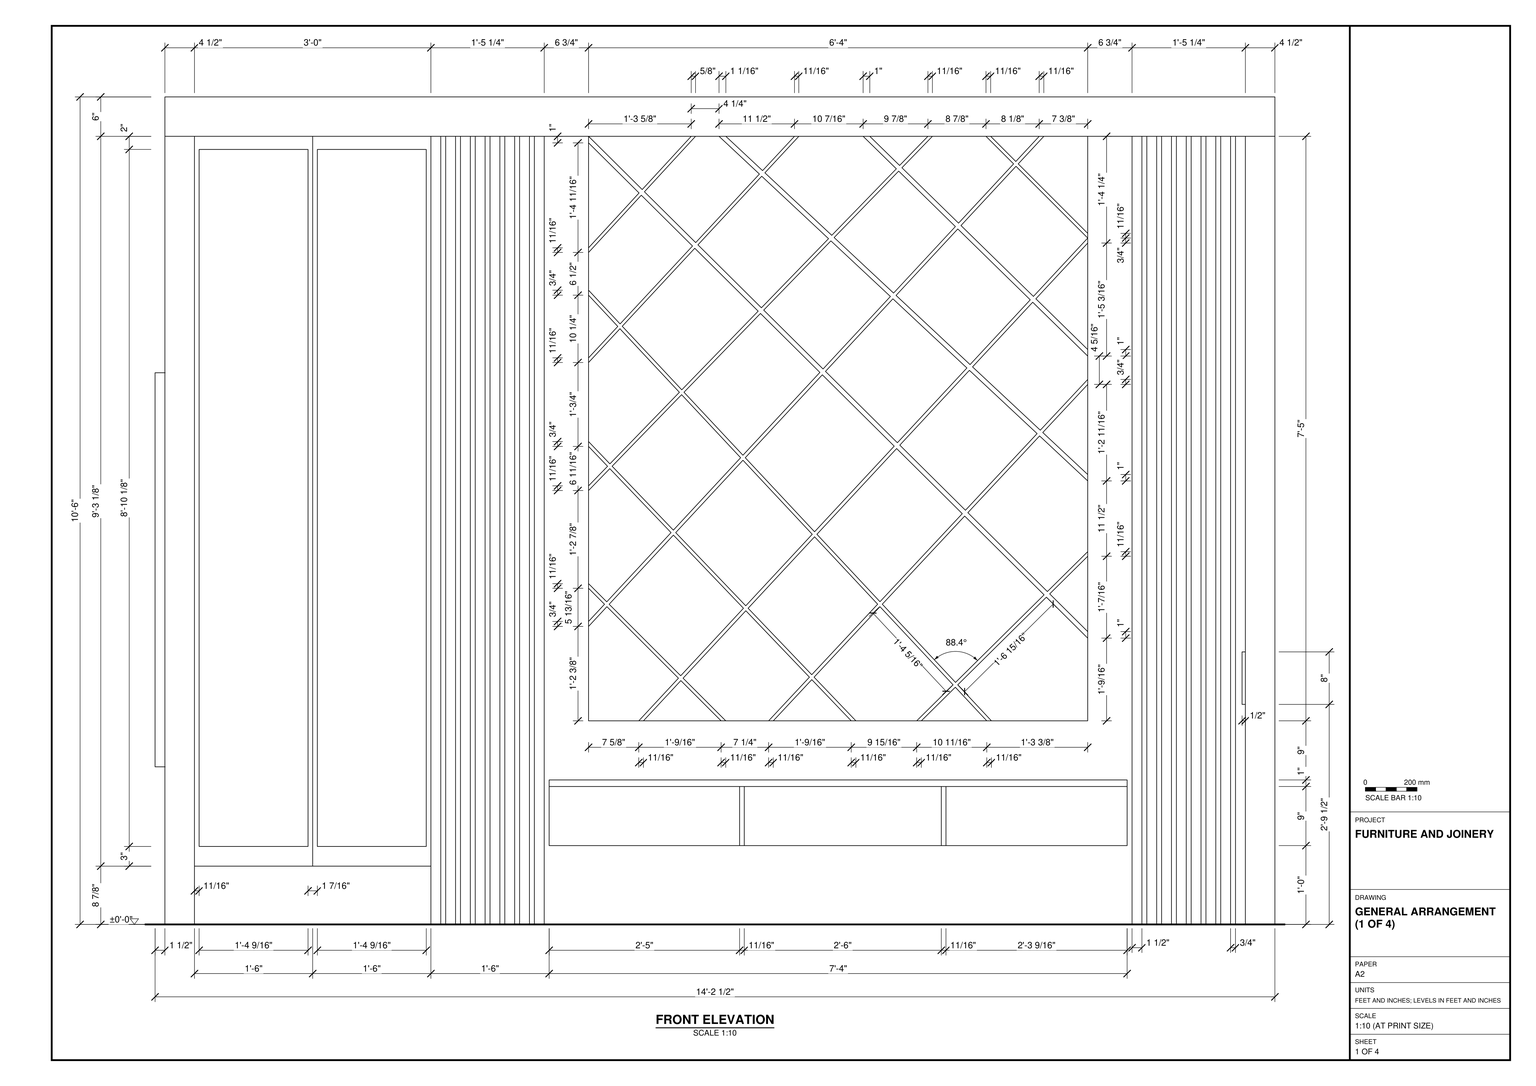
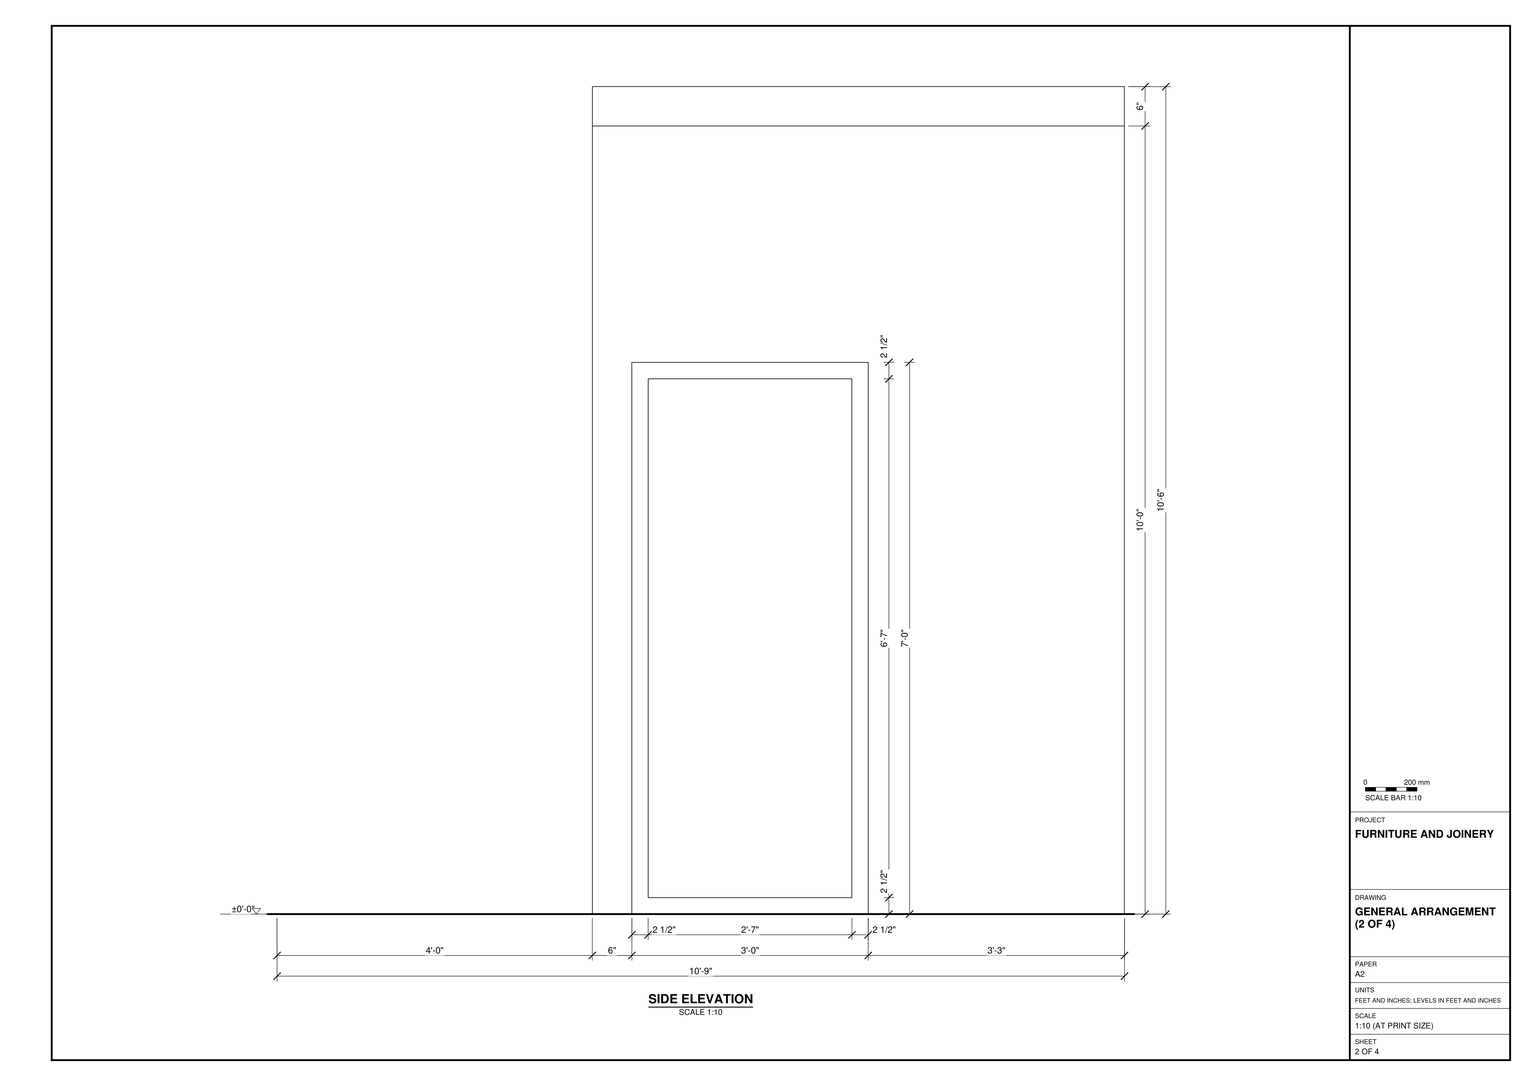
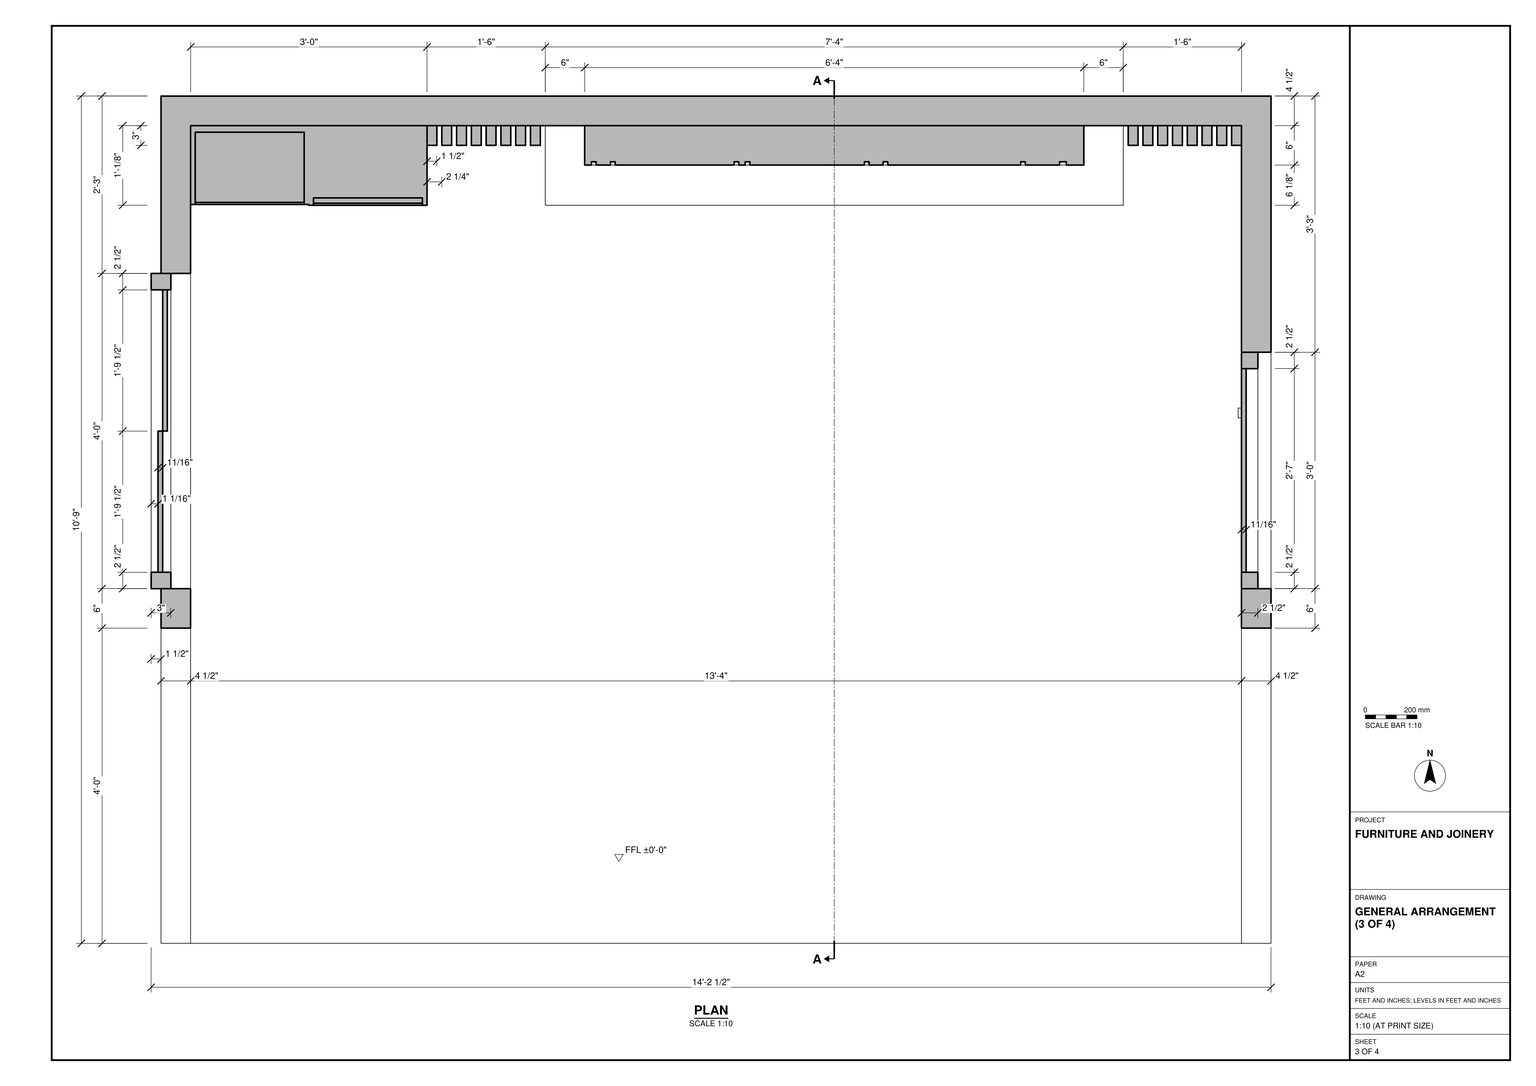
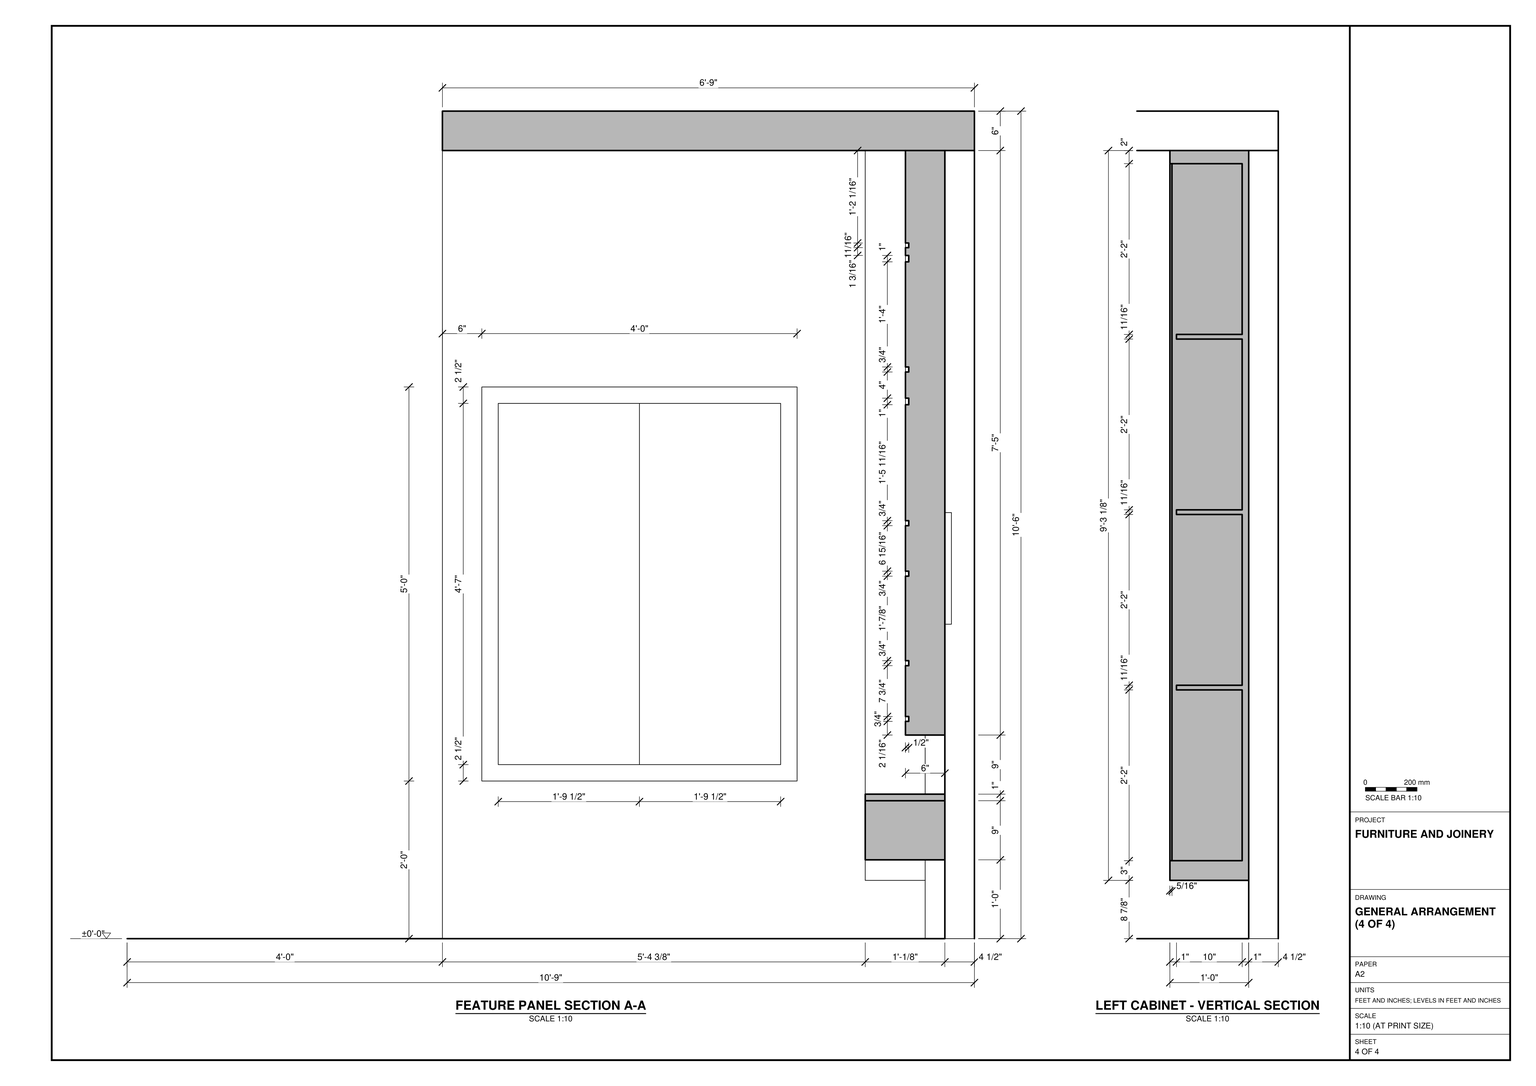
Build the feature-wall joinery and its surrounding room shell in SketchUp from task_files/diagram_01.pdf. Work in feet and inches. Set the finished floor at ±0'-0" and make the overall model 14'-2 1/2" wide, 10'-9" deep and 10'-6" high.

Use the plan to lay out the back wall and the two 4 1/2" thick side returns. Leave the front open, with the floor extending 4'-0" beyond the ends of the returns. Include the upper slab, the framed window in the left return and the framed door in the right return.

Facing the back wall, place the tall storage unit with paired inset fronts at the far left. Set out the central panel between the two bands of vertical slats. Follow the front elevation for the crossing diagonal lines, including where the diamonds are cut off at the panel edges. Below the panel, model the floating console with its thin top and three front sections. Use the plan to distinguish the projections of the panel, slats and storage units from the wall face.

Keep each shell element and each joinery piece in a separate group or component, and use components for repeated parts. Any decor or loose items shown may use suitable library components. Save one SketchUp model as output_files/feature_wall_with_built_in_storage_and_floating_console.skp.

# SketchUp Ruby script. Lengths in inches.
U = 1.inch
M = Sketchup.active_model
def pt(a) = Geom::Point3d.new(a.map { |v| v * U })
def face(e, loops, mat)
  f = e.add_face(loops[0].map { |a| pt(a) })
  loops[1..].each { |l| e.add_face(l.map { |a| pt(a) }).erase! }
  f.material = f.back_material = mat if mat
  f
end
# faces: each face lists its corners as indices into pts; further lists are holes
def faces(e, pts, list, mat = nil) = list.each { |f| face(e, (f[0].is_a?(Array) ? f : [f]).map { |l| l.map { |i| pts[i] } }, mat) }
# xy, xz, yz: faces in a plane at the given z, y or x. An outline is a flat list of corners, or four numbers for a rectangle; further outlines are holes
def ring(l) = l.size == 4 ? [[l[0], l[1]], [l[2], l[1]], [l[2], l[3]], [l[0], l[3]]] : l.each_slice(2).to_a
def flat(e, list, mat, &to3) = list.each { |f| face(e, (f[0].is_a?(Array) ? f : [f]).map { |l| ring(l).map { |u, v| to3.(u, v) } }, mat) }
def xy(e, z, list, mat = nil) = flat(e, list, mat) { |x, y| [x, y, z] }
def xz(e, y, list, mat = nil) = flat(e, list, mat) { |x, z| [x, y, z] }
def yz(e, x, list, mat = nil) = flat(e, list, mat) { |y, z| [x, y, z] }
def lines(e, pts, list) = list.each { |a, b| e.add_line(pt(pts[a]), pt(pts[b])) }
# prism: a flat outline (further loops are holes) pulled along v
def prism(e, loops, v, mat = nil)
  f = face(e, loops, mat); d = Geom::Vector3d.new(v.map { |x| x * U })
  f.pushpull(f.normal.samedirection?(d) ? d.length : -d.length)
end
def box(e, o, s, mat = nil) = prism(e, [[o, [o[0] + s[0], o[1], o[2]], [o[0] + s[0], o[1] + s[1], o[2]], [o[0], o[1] + s[1], o[2]]]], [0, 0, s[2]], mat)
def at(x, y, z, deg = 0) = Geom::Transformation.translation(pt([x, y, z])) * Geom::Transformation.rotation(ORIGIN, Z_AXIS, deg.degrees)
def axes(o, x, y, z) = Geom::Transformation.new([*x, 0, *y, 0, *z, 0, *pt(o).to_a, 1])
def part(name) = M.definitions.add(name)
# library, detail: a bought-in or finely detailed component or shape, given as its bounding box
def library(name, o, s) = part(name).tap { |d| box(d.entities, o, s) }
def detail(e, o, s) = box(e.add_group.entities, o, s)
def put(e, d, t, mat = nil) = e.add_instance(d, t).tap { |i| i.material = mat if mat }
def group(e, t, mat = nil) = e.add_group.tap { |g| g.transformation = t; g.material = mat if mat }.entities
root = M.entities
M.materials.add("Flooring Parquet Parallel E01 120cm").color = [119, 88, 63]
M.materials.add("Glass Yellow 001").color = [0, 0, 0]
M.materials["Glass Yellow 001"].alpha = 0.1
M.materials.add("Marble Beige 23-58 150cm").color = [206, 178, 147]
M.materials.add("Marble Black 01 150cm").color = [31, 31, 31]
M.materials.add("Metal Sandblasted Black 200cm").color = [86, 90, 95]
M.materials.add("Porcelain Poised Taupe Matte 001").color = [140, 135, 132]
M.materials.add("Wall Paint Fine Grain 01 Yellow 100cm").color = [207, 190, 139]
M.materials.add("Wood Tiles Dark Shiny 02 100cm").color = [42, 30, 20]
c1 = library("Group\#3",[0,-6,0],[76,6,89])
g1 = group(root,at(6,4.5,0))
xy(g1,0,[[0,-4.5,160,120]],"Marble Black 01 150cm")
xy(g1,0,[[-4.5,-4.5,0,43.5],[160,-4.5,164.5,43.5],[160,49.5,164.5,85.5]],"Porcelain Poised Taupe Matte 001")
xy(g1,24,[[-4.5,49.5,0,97.5]],"Wall Paint Fine Grain 01 Yellow 100cm")
xy(g1,84,[[160,49.5,164.5,85.5]],"Porcelain Poised Taupe Matte 001")
xy(g1,84,[[-4.5,49.5,0,97.5]],"Wall Paint Fine Grain 01 Yellow 100cm")
xy(g1,120,[[-4.5,43.5,0,43.5,0,120,160,120,160,43.5,164.5,43.5,164.5,124.5,-4.5,124.5]],"Porcelain Poised Taupe Matte 001")
xz(g1,43.5,[[-4.5,0,0,120],[160,0,164.5,120]],"Porcelain Poised Taupe Matte 001")
xz(g1,49.5,[[160,0,164.5,84]],"Porcelain Poised Taupe Matte 001")
xz(g1,49.5,[[-4.5,24,0,84]],"Wall Paint Fine Grain 01 Yellow 100cm")
xz(g1,85.5,[[160,0,164.5,84]],"Porcelain Poised Taupe Matte 001")
xz(g1,97.5,[[-4.5,24,0,84]],"Wall Paint Fine Grain 01 Yellow 100cm")
xz(g1,120,[[0,0,160,120]],"Porcelain Poised Taupe Matte 001")
xz(g1,121,[[18.71,47.875,35.29,64.875]])
xz(g1,124.5,[[-4.5,0,164.5,120]],"Porcelain Poised Taupe Matte 001")
yz(g1,-4.5,[[[43.5,0,124.5,120],[49.5,24,97.5,84]]],"Porcelain Poised Taupe Matte 001")
yz(g1,0,[[[43.5,0,120,120],[49.5,24,97.5,84]]],"Wall Paint Fine Grain 01 Yellow 100cm")
yz(g1,160,[[43.5,0,43.5,120,120,120,120,0,85.5,0,85.5,84,49.5,84,49.5,0]],"Wall Paint Fine Grain 01 Yellow 100cm")
yz(g1,164.5,[[43.5,0,49.5,0,49.5,84,85.5,84,85.5,0,124.5,0,124.5,120,43.5,120]],"Porcelain Poised Taupe Matte 001")
g2 = group(g1,at(-4.5,49.5,24))
xy(g2,0,[[-1.5,0,1.5,48]],"Metal Sandblasted Black 200cm")
xy(g2,2.5,[[-1.5,2.5,1.5,45.5]],"Metal Sandblasted Black 200cm")
xy(g2,57.5,[[-1.5,2.5,1.5,45.5]],"Metal Sandblasted Black 200cm")
xy(g2,60,[[-1.5,0,1.5,48]],"Metal Sandblasted Black 200cm")
xz(g2,0,[[-1.5,0,1.5,60]],"Metal Sandblasted Black 200cm")
xz(g2,2.5,[[-1.5,2.5,1.5,57.5]],"Metal Sandblasted Black 200cm")
xz(g2,45.5,[[-1.5,2.5,1.5,57.5]],"Metal Sandblasted Black 200cm")
xz(g2,48,[[-1.5,0,1.5,60]],"Metal Sandblasted Black 200cm")
yz(g2,-1.5,[[[0,0,48,60],[2.5,2.5,45.5,57.5]]],"Metal Sandblasted Black 200cm")
yz(g2,1.5,[[[0,0,48,60],[2.5,2.5,45.5,57.5]]],"Metal Sandblasted Black 200cm")
g3 = group(g2,at(0.25,24,2.5),"Glass Yellow 001")
box(g3,[0,0,0],[0.71,21.5,55])
g4 = group(g2,at(-0.46,2.5,2.5),"Glass Yellow 001")
box(g4,[0,0,0],[0.71,21.5,55])
g5 = group(g1,at(160,49.5,0))
xy(g5,0,[[0,0,2.5,36]])
xy(g5,2.5,[[0,2.5,2.5,33.5]])
xy(g5,81.5,[[0,2.5,2.5,33.5]])
xy(g5,84,[[0,0,2.5,36]])
xz(g5,0,[[0,0,2.5,84]])
xz(g5,2.5,[[0,2.5,2.5,81.5]])
xz(g5,33.5,[[0,2.5,2.5,81.5]])
xz(g5,36,[[0,0,2.5,84]])
yz(g5,0,[[[0,0,36,84],[2.5,2.5,33.5,81.5]]],"Metal Sandblasted Black 200cm")
yz(g5,2.5,[[[0,0,36,84],[2.5,2.5,33.5,81.5]]])
g6 = group(g5,at(0,2.5,2.5))
box(g6,[0,0,0],[0.71,31,79],"Wood Tiles Dark Shiny 02 100cm")
g7 = group(g6,at(0,25,31),"Metal Sandblasted Black 200cm")
xy(g7,0,[[-0.5,-1.5,0,0]])
xy(g7,8,[[-0.5,-1.5,0,0]])
xz(g7,-1.5,[[-0.5,0,0,8]])
xz(g7,0,[[-0.5,0,0,8]])
yz(g7,-0.5,[[-1.5,0,0,8]],"Metal Sandblasted Black 200cm")
yz(g7,0,[[-1.5,0,0,8]],"Metal Sandblasted Black 200cm")
g8 = group(root,at(6,124.5,0),"Porcelain Poised Taupe Matte 001")
xy(g8,8.875,[[18,-12.125,36,0],[0,-12,18,0]],"Porcelain Poised Taupe Matte 001")
xy(g8,11.875,[[18.71,-12.125,35.29,-1],[0.71,-12,17.29,-1]],"Porcelain Poised Taupe Matte 001")
xy(g8,29.46,[[18.71,-11,35.29,-1]],"Porcelain Poised Taupe Matte 001")
xy(g8,30.17,[[18.71,-11,35.29,-1]],"Porcelain Poised Taupe Matte 001")
xy(g8,37.875,[[0.71,-11,17.29,-1]],"Porcelain Poised Taupe Matte 001")
xy(g8,38.58,[[0.71,-11,17.29,-1]],"Porcelain Poised Taupe Matte 001")
xy(g8,47.17,[[18.71,-11,35.29,-1]],"Porcelain Poised Taupe Matte 001")
xy(g8,47.875,[[18.71,-11,35.29,1]],"Porcelain Poised Taupe Matte 001")
xy(g8,64.58,[[0.71,-11,17.29,-1]],"Porcelain Poised Taupe Matte 001")
xy(g8,64.875,[[18.71,-11,35.29,1]],"Porcelain Poised Taupe Matte 001")
xy(g8,65.29,[[0.71,-11,17.29,-1]],"Porcelain Poised Taupe Matte 001")
xy(g8,65.58,[[18.71,-11,35.29,0]],"Porcelain Poised Taupe Matte 001")
xy(g8,82.58,[[18.71,-11,35.29,0]],"Porcelain Poised Taupe Matte 001")
xy(g8,83.29,[[18.71,-11,35.29,0]],"Porcelain Poised Taupe Matte 001")
xy(g8,91.29,[[0.71,-11,17.29,-1]],"Porcelain Poised Taupe Matte 001")
xy(g8,92,[[0.71,-11,17.29,-1]],"Porcelain Poised Taupe Matte 001")
xy(g8,100.29,[[18.71,-11,35.29,0]],"Porcelain Poised Taupe Matte 001")
xy(g8,101,[[18.71,-11,35.29,0]],"Porcelain Poised Taupe Matte 001")
xy(g8,118,[[18.71,-12.125,35.29,0],[0.71,-12,17.29,-1]],"Porcelain Poised Taupe Matte 001")
xy(g8,120,[[18,-12.125,36,0],[0,-12,18,0]],"Porcelain Poised Taupe Matte 001")
xz(g8,-12.125,[[[18,8.875,36,120],[18.71,11.875,35.29,118]]],"Metal Sandblasted Black 200cm")
xz(g8,-12,[[[0,8.875,18,120],[0.71,11.875,17.29,118]]],"Metal Sandblasted Black 200cm")
xz(g8,-11,[[18.71,29.46,35.29,30.17],[0.71,37.875,17.29,38.58],[18.71,47.17,35.29,47.875],[0.71,64.58,17.29,65.29],[18.71,64.875,35.29,65.58],
  [18.71,82.58,35.29,83.29],[0.71,91.29,17.29,92],[18.71,100.29,35.29,101]],"Porcelain Poised Taupe Matte 001")
xz(g8,-1,[[0.71,11.875,17.29,37.875],[18.71,11.875,35.29,29.46],[18.71,30.17,35.29,47.17],[0.71,38.58,17.29,64.58],[0.71,65.29,17.29,91.29],
  [0.71,92,17.29,118]],"Porcelain Poised Taupe Matte 001")
xz(g8,0,[[18.71,65.58,35.29,82.58],[18.71,83.29,35.29,100.29],[18.71,101,35.29,118]],"Porcelain Poised Taupe Matte 001")
xz(g8,1,[[18.71,47.875,35.29,64.875]],"Porcelain Poised Taupe Matte 001")
yz(g8,0,[[-12,8.875,0,120]],"Porcelain Poised Taupe Matte 001")
yz(g8,0.71,[[-12,11.875,-1,11.875,-1,37.875,-11,37.875,-11,38.58,-1,38.58,-1,64.58,-11,64.58,-11,65.29,-1,65.29,-1,91.29,-11,91.29,-11,92,-1,92,-1,118,-12,118]],"Porcelain Poised Taupe Matte 001")
yz(g8,17.29,[[-12,11.875,-12,118,-1,118,-1,92,-11,92,-11,91.29,-1,91.29,-1,65.29,-11,65.29,-11,64.58,-1,64.58,-1,38.58,-11,38.58,-11,37.875,-1,37.875,-1,11.875]],"Porcelain Poised Taupe Matte 001")
yz(g8,18,[[-12.125,8.875,-12,120]],"Porcelain Poised Taupe Matte 001")
yz(g8,18.71,[[-12.125,11.875,-1,11.875,-1,29.46,-11,29.46,-11,30.17,-1,30.17,-1,47.17,-11,47.17,-11,47.875,1,47.875,1,64.875,-11,64.875,-11,65.58,0,65.58,0,82.58,-11,82.58,-11,83.29,0,83.29,0,100.29,-11,100.29,-11,101,0,101,0,118,-12.125,118]],"Porcelain Poised Taupe Matte 001")
yz(g8,35.29,[[-12.125,11.875,-12.125,118,0,118,0,101,-11,101,-11,100.29,0,100.29,0,83.29,-11,83.29,-11,82.58,0,82.58,0,65.58,-11,65.58,-11,64.875,1,64.875,1,47.875,-11,47.875,-11,47.17,-1,47.17,-1,30.17,-11,30.17,-11,29.46,-1,29.46,-1,11.875]],"Porcelain Poised Taupe Matte 001")
yz(g8,36,[[-12.125,8.875,0,120]],"Porcelain Poised Taupe Matte 001")
p = [[0,0,0],[0,0,8.17],[36,0,0],[0,0,8.875],[-0.35,0,8.17]]
lines(g8,p,[[0,1],[2,0],[1,3],[1,4]])
g9 = group(g8,at(0.71,-12,11.875),"Glass Yellow 001")
box(g9,[0,0,0],[16.58,0.31,106.125])
g10 = group(g8,at(18.71,-12.125,11.875),"Glass Yellow 001")
box(g10,[0,0,0],[16.58,0.31,106.125])
put(root,c1,at(66,124.5,31),"Marble Beige 23-58 150cm")
g11 = group(root,at(60,124.5,12))
xy(g11,0,[[0,-12.125,0,0,88,0,88,-12.125,60.42,-12.125,60.42,-11.625,59.71,-11.625,59.71,-12.125,29.71,-12.125,29.71,-11.625,29,-11.625,29,-12.125]])
xy(g11,9,[[0,-12.125,29,-12.125,29,-11.625,29.71,-11.625,29.71,-12.125,59.71,-12.125,59.71,-11.625,60.42,-11.625,60.42,-12.125,88,-12.125,88,0,0,0]])
xz(g11,-12.125,[[0,0,29,9],[29.71,0,59.71,9],[60.42,0,88,9]])
xz(g11,-11.625,[[29,0,29.71,9],[59.71,0,60.42,9]],"Metal Sandblasted Black 200cm")
xz(g11,0,[[0,0,88,9]])
yz(g11,0,[[-12.125,0,0,9]])
yz(g11,29,[[-12.125,0,-11.625,9]])
yz(g11,29.71,[[-12.125,0,-11.625,9]])
yz(g11,59.71,[[-12.125,0,-11.625,9]])
yz(g11,60.42,[[-12.125,0,-11.625,9]])
yz(g11,88,[[-12.125,0,0,9]])
g12 = group(root,at(60,124.5,21),"Marble Black 01 150cm")
box(g12,[0,-12.125,0],[88,12.125,1],"Marble Black 01 150cm")
g13 = group(root,at(42,124.5,0),"Flooring Parquet Parallel E01 120cm")
box(g13,[0,-3,0],[1.5,3,120],"Flooring Parquet Parallel E01 120cm")
g14 = group(root,at(44.25,124.5,0),"Flooring Parquet Parallel E01 120cm")
box(g14,[0,-3,0],[1.5,3,120],"Flooring Parquet Parallel E01 120cm")
g15 = group(root,at(46.5,124.5,0),"Flooring Parquet Parallel E01 120cm")
box(g15,[0,-3,0],[1.5,3,120],"Flooring Parquet Parallel E01 120cm")
g16 = group(root,at(48.75,124.5,0),"Flooring Parquet Parallel E01 120cm")
box(g16,[0,-3,0],[1.5,3,120],"Flooring Parquet Parallel E01 120cm")
g17 = group(root,at(51,124.5,0),"Flooring Parquet Parallel E01 120cm")
box(g17,[0,-3,0],[1.5,3,120],"Flooring Parquet Parallel E01 120cm")
g18 = group(root,at(53.25,124.5,0),"Flooring Parquet Parallel E01 120cm")
box(g18,[0,-3,0],[1.5,3,120],"Flooring Parquet Parallel E01 120cm")
g19 = group(root,at(55.5,124.5,0),"Flooring Parquet Parallel E01 120cm")
box(g19,[0,-3,0],[1.5,3,120],"Flooring Parquet Parallel E01 120cm")
g20 = group(root,at(57.75,124.5,0),"Flooring Parquet Parallel E01 120cm")
box(g20,[0,-3,0],[1.5,3,120],"Flooring Parquet Parallel E01 120cm")
g21 = group(root,at(164.5,124.5,0),"Flooring Parquet Parallel E01 120cm")
box(g21,[0,-3,0],[1.5,3,120],"Flooring Parquet Parallel E01 120cm")
g22 = group(root,at(162.25,124.5,0),"Flooring Parquet Parallel E01 120cm")
box(g22,[0,-3,0],[1.5,3,120],"Flooring Parquet Parallel E01 120cm")
g23 = group(root,at(160,124.5,0),"Flooring Parquet Parallel E01 120cm")
box(g23,[0,-3,0],[1.5,3,120],"Flooring Parquet Parallel E01 120cm")
g24 = group(root,at(157.75,124.5,0),"Flooring Parquet Parallel E01 120cm")
box(g24,[0,-3,0],[1.5,3,120],"Flooring Parquet Parallel E01 120cm")
g25 = group(root,at(155.5,124.5,0),"Flooring Parquet Parallel E01 120cm")
box(g25,[0,-3,0],[1.5,3,120],"Flooring Parquet Parallel E01 120cm")
g26 = group(root,at(153.25,124.5,0),"Flooring Parquet Parallel E01 120cm")
box(g26,[0,-3,0],[1.5,3,120],"Flooring Parquet Parallel E01 120cm")
g27 = group(root,at(151,124.5,0),"Flooring Parquet Parallel E01 120cm")
box(g27,[0,-3,0],[1.5,3,120],"Flooring Parquet Parallel E01 120cm")
g28 = group(root,at(148.75,124.5,0),"Flooring Parquet Parallel E01 120cm")
box(g28,[0,-3,0],[1.5,3,120],"Flooring Parquet Parallel E01 120cm")
g29 = group(root,at(1.5,48,120))
box(g29,[0,0,0],[169,81,6])
